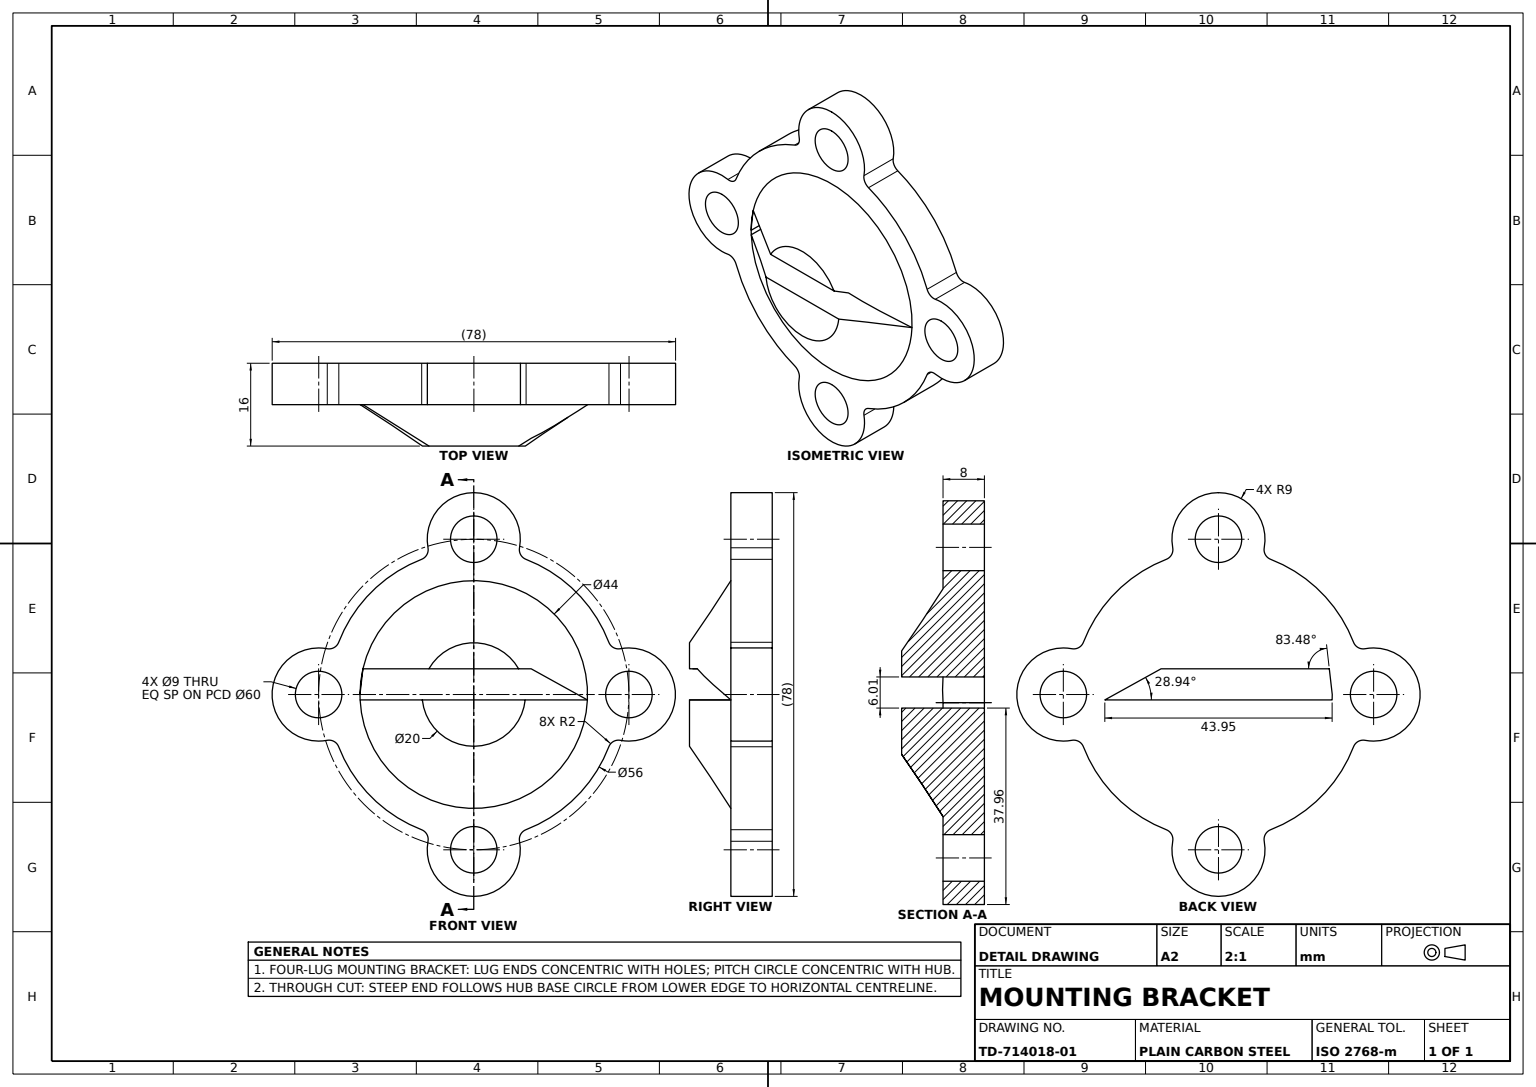
ISO-10303-21;
HEADER;
FILE_DESCRIPTION((''),'2;1');
FILE_NAME('','',(''),(''),'','','');
FILE_SCHEMA(('AUTOMOTIVE_DESIGN'));
ENDSEC;
DATA;
#1=APPLICATION_CONTEXT('');
#2=PRODUCT_CONTEXT('',#1,'mechanical');
#3=PRODUCT('','','',(#2));
#4=PRODUCT_DEFINITION_FORMATION('','',#3);
#5=PRODUCT_DEFINITION_CONTEXT('',#1,'design');
#6=PRODUCT_DEFINITION('','',#4,#5);
#7=PRODUCT_DEFINITION_SHAPE('','',#6);
#8=(LENGTH_UNIT()NAMED_UNIT(*)SI_UNIT(.MILLI.,.METRE.));
#9=(NAMED_UNIT(*)PLANE_ANGLE_UNIT()SI_UNIT($,.RADIAN.));
#10=(NAMED_UNIT(*)SI_UNIT($,.STERADIAN.)SOLID_ANGLE_UNIT());
#11=UNCERTAINTY_MEASURE_WITH_UNIT(LENGTH_MEASURE(1.E-05),#8,'distance_accuracy_value','');
#12=(GEOMETRIC_REPRESENTATION_CONTEXT(3)GLOBAL_UNCERTAINTY_ASSIGNED_CONTEXT((#11))GLOBAL_UNIT_ASSIGNED_CONTEXT((#8,#9,#10))REPRESENTATION_CONTEXT('',''));
#13=CARTESIAN_POINT('',(30.,0.,9.));
#14=VERTEX_POINT('',#13);
#15=CARTESIAN_POINT('',(30.,0.,-9.));
#16=VERTEX_POINT('',#15);
#17=CARTESIAN_POINT('',(30.,0.,0.));
#18=DIRECTION('',(0.,1.,0.));
#19=DIRECTION('',(0.,0.,1.));
#20=AXIS2_PLACEMENT_3D('',#17,#18,#19);
#21=CIRCLE('',#20,9.);
#22=EDGE_CURVE('',#14,#16,#21,.T.);
#23=ORIENTED_EDGE('',*,*,#22,.T.);
#24=CARTESIAN_POINT('',(30.,8.,-9.));
#25=VERTEX_POINT('',#24);
#26=DIRECTION('',(0.,-1.,0.));
#27=VECTOR('',#26,1000.);
#28=LINE('',#24,#27);
#29=EDGE_CURVE('',#25,#16,#28,.T.);
#30=ORIENTED_EDGE('',*,*,#29,.F.);
#31=CARTESIAN_POINT('',(30.,8.,9.));
#32=VERTEX_POINT('',#31);
#33=CARTESIAN_POINT('',(30.,8.,0.));
#34=AXIS2_PLACEMENT_3D('',#33,#18,#19);
#35=CIRCLE('',#34,9.);
#36=EDGE_CURVE('',#32,#25,#35,.T.);
#37=ORIENTED_EDGE('',*,*,#36,.F.);
#38=LINE('',#31,#27);
#39=EDGE_CURVE('',#32,#14,#38,.T.);
#40=ORIENTED_EDGE('',*,*,#39,.T.);
#41=EDGE_LOOP('',(#23,#30,#37,#40));
#42=FACE_OUTER_BOUND('',#41,.T.);
#43=DIRECTION('',(0.,0.,-1.));
#44=AXIS2_PLACEMENT_3D('',#33,#26,#43);
#45=CYLINDRICAL_SURFACE('',#44,9.);
#46=ADVANCED_FACE('',(#42),#45,.T.);
#47=CARTESIAN_POINT('',(-28.35,8.,-8.847457));
#48=VERTEX_POINT('',#47);
#49=CARTESIAN_POINT('',(-30.,8.,-9.));
#50=VERTEX_POINT('',#49);
#51=CARTESIAN_POINT('',(-30.,8.,0.));
#52=AXIS2_PLACEMENT_3D('',#51,#18,#19);
#53=CIRCLE('',#52,9.);
#54=EDGE_CURVE('',#48,#50,#53,.T.);
#55=ORIENTED_EDGE('',*,*,#54,.F.);
#56=CARTESIAN_POINT('',(-28.35,0.,-8.847457));
#57=VERTEX_POINT('',#56);
#58=LINE('',#47,#27);
#59=EDGE_CURVE('',#48,#57,#58,.T.);
#60=ORIENTED_EDGE('',*,*,#59,.T.);
#61=CARTESIAN_POINT('',(-30.,0.,-9.));
#62=VERTEX_POINT('',#61);
#63=CARTESIAN_POINT('',(-30.,0.,0.));
#64=AXIS2_PLACEMENT_3D('',#63,#18,#19);
#65=CIRCLE('',#64,9.);
#66=EDGE_CURVE('',#57,#62,#65,.T.);
#67=ORIENTED_EDGE('',*,*,#66,.T.);
#68=LINE('',#49,#27);
#69=EDGE_CURVE('',#50,#62,#68,.T.);
#70=ORIENTED_EDGE('',*,*,#69,.F.);
#71=EDGE_LOOP('',(#55,#60,#67,#70));
#72=FACE_OUTER_BOUND('',#71,.T.);
#73=AXIS2_PLACEMENT_3D('',#51,#26,#43);
#74=CYLINDRICAL_SURFACE('',#73,9.);
#75=ADVANCED_FACE('',(#72),#74,.T.);
#76=CARTESIAN_POINT('',(-8.847457,8.,-28.35));
#77=VERTEX_POINT('',#76);
#78=CARTESIAN_POINT('',(-8.847457,0.,-28.35));
#79=VERTEX_POINT('',#78);
#80=LINE('',#76,#27);
#81=EDGE_CURVE('',#77,#79,#80,.T.);
#82=ORIENTED_EDGE('',*,*,#81,.F.);
#83=CARTESIAN_POINT('',(0.,8.,-39.));
#84=VERTEX_POINT('',#83);
#85=CARTESIAN_POINT('',(0.,8.,-30.));
#86=AXIS2_PLACEMENT_3D('',#85,#18,#19);
#87=CIRCLE('',#86,9.);
#88=EDGE_CURVE('',#84,#77,#87,.T.);
#89=ORIENTED_EDGE('',*,*,#88,.F.);
#90=CARTESIAN_POINT('',(0.,0.,-39.));
#91=VERTEX_POINT('',#90);
#92=LINE('',#83,#27);
#93=EDGE_CURVE('',#84,#91,#92,.T.);
#94=ORIENTED_EDGE('',*,*,#93,.T.);
#95=CARTESIAN_POINT('',(0.,0.,-30.));
#96=AXIS2_PLACEMENT_3D('',#95,#18,#19);
#97=CIRCLE('',#96,9.);
#98=EDGE_CURVE('',#91,#79,#97,.T.);
#99=ORIENTED_EDGE('',*,*,#98,.T.);
#100=EDGE_LOOP('',(#82,#89,#94,#99));
#101=FACE_OUTER_BOUND('',#100,.T.);
#102=AXIS2_PLACEMENT_3D('',#85,#26,#43);
#103=CYLINDRICAL_SURFACE('',#102,9.);
#104=ADVANCED_FACE('',(#101),#103,.T.);
#105=CARTESIAN_POINT('',(-10.092655,8.,26.117778));
#106=VERTEX_POINT('',#105);
#107=CARTESIAN_POINT('',(-10.092655,0.,26.117778));
#108=VERTEX_POINT('',#107);
#109=LINE('',#105,#27);
#110=EDGE_CURVE('',#106,#108,#109,.T.);
#111=ORIENTED_EDGE('',*,*,#110,.F.);
#112=CARTESIAN_POINT('',(-26.117778,8.,10.092655));
#113=VERTEX_POINT('',#112);
#114=CARTESIAN_POINT('',(0.,8.,0.));
#115=AXIS2_PLACEMENT_3D('',#114,#18,#19);
#116=CIRCLE('',#115,28.);
#117=EDGE_CURVE('',#113,#106,#116,.T.);
#118=ORIENTED_EDGE('',*,*,#117,.F.);
#119=CARTESIAN_POINT('',(-26.117778,0.,10.092655));
#120=VERTEX_POINT('',#119);
#121=LINE('',#112,#27);
#122=EDGE_CURVE('',#113,#120,#121,.T.);
#123=ORIENTED_EDGE('',*,*,#122,.T.);
#124=CARTESIAN_POINT('',(0.,0.,0.));
#125=AXIS2_PLACEMENT_3D('',#124,#18,#19);
#126=CIRCLE('',#125,28.);
#127=EDGE_CURVE('',#120,#108,#126,.T.);
#128=ORIENTED_EDGE('',*,*,#127,.T.);
#129=EDGE_LOOP('',(#111,#118,#123,#128));
#130=FACE_OUTER_BOUND('',#129,.T.);
#131=AXIS2_PLACEMENT_3D('',#114,#26,#43);
#132=CYLINDRICAL_SURFACE('',#131,28.);
#133=ADVANCED_FACE('',(#130),#132,.T.);
#134=CARTESIAN_POINT('',(26.117778,0.,10.092655));
#135=VERTEX_POINT('',#134);
#136=CARTESIAN_POINT('',(27.983333,0.,8.813559));
#137=VERTEX_POINT('',#136);
#138=CARTESIAN_POINT('',(27.983333,0.,10.813559));
#139=AXIS2_PLACEMENT_3D('',#138,#26,#43);
#140=CIRCLE('',#139,2.);
#141=EDGE_CURVE('',#135,#137,#140,.T.);
#142=ORIENTED_EDGE('',*,*,#141,.T.);
#143=CARTESIAN_POINT('',(27.983333,8.,8.813559));
#144=VERTEX_POINT('',#143);
#145=LINE('',#143,#27);
#146=EDGE_CURVE('',#144,#137,#145,.T.);
#147=ORIENTED_EDGE('',*,*,#146,.F.);
#148=CARTESIAN_POINT('',(26.117778,8.,10.092655));
#149=VERTEX_POINT('',#148);
#150=CARTESIAN_POINT('',(27.983333,8.,10.813559));
#151=AXIS2_PLACEMENT_3D('',#150,#26,#43);
#152=CIRCLE('',#151,2.);
#153=EDGE_CURVE('',#149,#144,#152,.T.);
#154=ORIENTED_EDGE('',*,*,#153,.F.);
#155=LINE('',#148,#27);
#156=EDGE_CURVE('',#149,#135,#155,.T.);
#157=ORIENTED_EDGE('',*,*,#156,.T.);
#158=EDGE_LOOP('',(#142,#147,#154,#157));
#159=FACE_OUTER_BOUND('',#158,.T.);
#160=CYLINDRICAL_SURFACE('',#151,2.);
#161=ADVANCED_FACE('',(#159),#160,.F.);
#162=CARTESIAN_POINT('',(30.,8.,4.5));
#163=VERTEX_POINT('',#162);
#164=CARTESIAN_POINT('',(30.,0.,4.5));
#165=VERTEX_POINT('',#164);
#166=LINE('',#162,#27);
#167=EDGE_CURVE('',#163,#165,#166,.T.);
#168=ORIENTED_EDGE('',*,*,#167,.T.);
#169=CARTESIAN_POINT('',(30.,0.,-4.5));
#170=VERTEX_POINT('',#169);
#171=CIRCLE('',#20,4.5);
#172=EDGE_CURVE('',#170,#165,#171,.T.);
#173=ORIENTED_EDGE('',*,*,#172,.F.);
#174=CARTESIAN_POINT('',(30.,8.,-4.5));
#175=VERTEX_POINT('',#174);
#176=LINE('',#174,#27);
#177=EDGE_CURVE('',#175,#170,#176,.T.);
#178=ORIENTED_EDGE('',*,*,#177,.F.);
#179=CIRCLE('',#34,4.5);
#180=EDGE_CURVE('',#175,#163,#179,.T.);
#181=ORIENTED_EDGE('',*,*,#180,.T.);
#182=EDGE_LOOP('',(#168,#173,#178,#181));
#183=FACE_OUTER_BOUND('',#182,.T.);
#184=CYLINDRICAL_SURFACE('',#44,4.5);
#185=ADVANCED_FACE('',(#183),#184,.F.);
#186=CARTESIAN_POINT('',(8.678873,16.,-4.967612));
#187=VERTEX_POINT('',#186);
#188=CARTESIAN_POINT('',(-8.678875,16.,-4.967612));
#189=VERTEX_POINT('',#188);
#190=CARTESIAN_POINT('',(0.,16.,0.));
#191=AXIS2_PLACEMENT_3D('',#190,#18,#19);
#192=CIRCLE('',#191,10.);
#193=EDGE_CURVE('',#187,#189,#192,.T.);
#194=ORIENTED_EDGE('',*,*,#193,.T.);
#195=CARTESIAN_POINT('',(0.,16.,-4.967612));
#196=DIRECTION('',(-1.,0.,0.));
#197=VECTOR('',#196,1000.);
#198=LINE('',#195,#197);
#199=EDGE_CURVE('',#187,#189,#198,.T.);
#200=ORIENTED_EDGE('',*,*,#199,.F.);
#201=EDGE_LOOP('',(#194,#200));
#202=FACE_OUTER_BOUND('',#201,.T.);
#203=PLANE('',#191);
#204=ADVANCED_FACE('',(#202),#203,.T.);
#205=CARTESIAN_POINT('',(-30.,8.,4.5));
#206=VERTEX_POINT('',#205);
#207=CARTESIAN_POINT('',(-30.,0.,4.5));
#208=VERTEX_POINT('',#207);
#209=LINE('',#205,#27);
#210=EDGE_CURVE('',#206,#208,#209,.T.);
#211=ORIENTED_EDGE('',*,*,#210,.F.);
#212=CARTESIAN_POINT('',(-30.,8.,-4.5));
#213=VERTEX_POINT('',#212);
#214=CIRCLE('',#52,4.5);
#215=EDGE_CURVE('',#206,#213,#214,.T.);
#216=ORIENTED_EDGE('',*,*,#215,.T.);
#217=CARTESIAN_POINT('',(-30.,0.,-4.5));
#218=VERTEX_POINT('',#217);
#219=LINE('',#212,#27);
#220=EDGE_CURVE('',#213,#218,#219,.T.);
#221=ORIENTED_EDGE('',*,*,#220,.T.);
#222=CIRCLE('',#64,4.5);
#223=EDGE_CURVE('',#208,#218,#222,.T.);
#224=ORIENTED_EDGE('',*,*,#223,.F.);
#225=EDGE_LOOP('',(#211,#216,#221,#224));
#226=FACE_OUTER_BOUND('',#225,.T.);
#227=CYLINDRICAL_SURFACE('',#73,4.5);
#228=ADVANCED_FACE('',(#226),#227,.F.);
#229=CARTESIAN_POINT('',(10.092655,8.,-26.117778));
#230=VERTEX_POINT('',#229);
#231=CARTESIAN_POINT('',(10.092655,0.,-26.117778));
#232=VERTEX_POINT('',#231);
#233=LINE('',#229,#27);
#234=EDGE_CURVE('',#230,#232,#233,.T.);
#235=ORIENTED_EDGE('',*,*,#234,.F.);
#236=CARTESIAN_POINT('',(26.117778,8.,-10.092655));
#237=VERTEX_POINT('',#236);
#238=EDGE_CURVE('',#237,#230,#116,.T.);
#239=ORIENTED_EDGE('',*,*,#238,.F.);
#240=CARTESIAN_POINT('',(26.117778,0.,-10.092655));
#241=VERTEX_POINT('',#240);
#242=LINE('',#236,#27);
#243=EDGE_CURVE('',#237,#241,#242,.T.);
#244=ORIENTED_EDGE('',*,*,#243,.T.);
#245=EDGE_CURVE('',#241,#232,#126,.T.);
#246=ORIENTED_EDGE('',*,*,#245,.T.);
#247=EDGE_LOOP('',(#235,#239,#244,#246));
#248=FACE_OUTER_BOUND('',#247,.T.);
#249=ADVANCED_FACE('',(#248),#132,.T.);
#250=CARTESIAN_POINT('',(0.,0.,34.5));
#251=VERTEX_POINT('',#250);
#252=CARTESIAN_POINT('',(0.,0.,25.5));
#253=VERTEX_POINT('',#252);
#254=CARTESIAN_POINT('',(0.,0.,30.));
#255=AXIS2_PLACEMENT_3D('',#254,#18,#19);
#256=CIRCLE('',#255,4.5);
#257=EDGE_CURVE('',#251,#253,#256,.T.);
#258=ORIENTED_EDGE('',*,*,#257,.F.);
#259=CARTESIAN_POINT('',(0.,8.,34.5));
#260=VERTEX_POINT('',#259);
#261=LINE('',#259,#27);
#262=EDGE_CURVE('',#260,#251,#261,.T.);
#263=ORIENTED_EDGE('',*,*,#262,.F.);
#264=CARTESIAN_POINT('',(0.,8.,25.5));
#265=VERTEX_POINT('',#264);
#266=CARTESIAN_POINT('',(0.,8.,30.));
#267=AXIS2_PLACEMENT_3D('',#266,#18,#19);
#268=CIRCLE('',#267,4.5);
#269=EDGE_CURVE('',#260,#265,#268,.T.);
#270=ORIENTED_EDGE('',*,*,#269,.T.);
#271=LINE('',#264,#27);
#272=EDGE_CURVE('',#265,#253,#271,.T.);
#273=ORIENTED_EDGE('',*,*,#272,.T.);
#274=EDGE_LOOP('',(#258,#263,#270,#273));
#275=FACE_OUTER_BOUND('',#274,.T.);
#276=AXIS2_PLACEMENT_3D('',#266,#26,#43);
#277=CYLINDRICAL_SURFACE('',#276,4.5);
#278=ADVANCED_FACE('',(#275),#277,.F.);
#279=CARTESIAN_POINT('',(-30.,8.,9.));
#280=VERTEX_POINT('',#279);
#281=EDGE_CURVE('',#50,#280,#53,.T.);
#282=ORIENTED_EDGE('',*,*,#281,.F.);
#283=ORIENTED_EDGE('',*,*,#69,.T.);
#284=CARTESIAN_POINT('',(-30.,0.,9.));
#285=VERTEX_POINT('',#284);
#286=EDGE_CURVE('',#62,#285,#65,.T.);
#287=ORIENTED_EDGE('',*,*,#286,.T.);
#288=LINE('',#279,#27);
#289=EDGE_CURVE('',#280,#285,#288,.T.);
#290=ORIENTED_EDGE('',*,*,#289,.F.);
#291=EDGE_LOOP('',(#282,#283,#287,#290));
#292=FACE_OUTER_BOUND('',#291,.T.);
#293=ADVANCED_FACE('',(#292),#74,.T.);
#294=CARTESIAN_POINT('',(0.,8.,-34.5));
#295=VERTEX_POINT('',#294);
#296=CARTESIAN_POINT('',(0.,8.,-25.5));
#297=VERTEX_POINT('',#296);
#298=CIRCLE('',#86,4.5);
#299=EDGE_CURVE('',#295,#297,#298,.T.);
#300=ORIENTED_EDGE('',*,*,#299,.T.);
#301=CARTESIAN_POINT('',(0.,0.,-25.5));
#302=VERTEX_POINT('',#301);
#303=LINE('',#296,#27);
#304=EDGE_CURVE('',#297,#302,#303,.T.);
#305=ORIENTED_EDGE('',*,*,#304,.T.);
#306=CARTESIAN_POINT('',(0.,0.,-34.5));
#307=VERTEX_POINT('',#306);
#308=CIRCLE('',#96,4.5);
#309=EDGE_CURVE('',#307,#302,#308,.T.);
#310=ORIENTED_EDGE('',*,*,#309,.F.);
#311=LINE('',#294,#27);
#312=EDGE_CURVE('',#295,#307,#311,.T.);
#313=ORIENTED_EDGE('',*,*,#312,.F.);
#314=EDGE_LOOP('',(#300,#305,#310,#313));
#315=FACE_OUTER_BOUND('',#314,.T.);
#316=CYLINDRICAL_SURFACE('',#102,4.5);
#317=ADVANCED_FACE('',(#315),#316,.F.);
#318=CARTESIAN_POINT('',(-9.945407,16.,1.043517));
#319=VERTEX_POINT('',#318);
#320=CARTESIAN_POINT('',(8.632899,16.,5.047085));
#321=VERTEX_POINT('',#320);
#322=EDGE_CURVE('',#319,#321,#192,.T.);
#323=ORIENTED_EDGE('',*,*,#322,.T.);
#324=CARTESIAN_POINT('',(9.945404,16.,1.043517));
#325=VERTEX_POINT('',#324);
#326=EDGE_CURVE('',#321,#325,#192,.T.);
#327=ORIENTED_EDGE('',*,*,#326,.T.);
#328=CARTESIAN_POINT('',(0.,16.,1.043517));
#329=DIRECTION('',(1.,0.,0.));
#330=VECTOR('',#329,1000.);
#331=LINE('',#328,#330);
#332=EDGE_CURVE('',#319,#325,#331,.T.);
#333=ORIENTED_EDGE('',*,*,#332,.F.);
#334=EDGE_LOOP('',(#323,#327,#333));
#335=FACE_OUTER_BOUND('',#334,.T.);
#336=ADVANCED_FACE('',(#335),#203,.T.);
#337=CARTESIAN_POINT('',(28.35,8.,-8.847457));
#338=VERTEX_POINT('',#337);
#339=CARTESIAN_POINT('',(28.35,0.,-8.847457));
#340=VERTEX_POINT('',#339);
#341=LINE('',#337,#27);
#342=EDGE_CURVE('',#338,#340,#341,.T.);
#343=ORIENTED_EDGE('',*,*,#342,.T.);
#344=CARTESIAN_POINT('',(27.983333,0.,-10.813559));
#345=AXIS2_PLACEMENT_3D('',#344,#26,#19);
#346=CIRCLE('',#345,2.);
#347=EDGE_CURVE('',#340,#241,#346,.T.);
#348=ORIENTED_EDGE('',*,*,#347,.T.);
#349=ORIENTED_EDGE('',*,*,#243,.F.);
#350=CARTESIAN_POINT('',(27.983333,8.,-10.813559));
#351=AXIS2_PLACEMENT_3D('',#350,#26,#19);
#352=CIRCLE('',#351,2.);
#353=EDGE_CURVE('',#338,#237,#352,.T.);
#354=ORIENTED_EDGE('',*,*,#353,.F.);
#355=EDGE_LOOP('',(#343,#348,#349,#354));
#356=FACE_OUTER_BOUND('',#355,.T.);
#357=AXIS2_PLACEMENT_3D('',#350,#26,#43);
#358=CYLINDRICAL_SURFACE('',#357,2.);
#359=ADVANCED_FACE('',(#356),#358,.F.);
#360=EDGE_CURVE('',#163,#175,#179,.T.);
#361=ORIENTED_EDGE('',*,*,#360,.T.);
#362=ORIENTED_EDGE('',*,*,#177,.T.);
#363=EDGE_CURVE('',#165,#170,#171,.T.);
#364=ORIENTED_EDGE('',*,*,#363,.F.);
#365=ORIENTED_EDGE('',*,*,#167,.F.);
#366=EDGE_LOOP('',(#361,#362,#364,#365));
#367=FACE_OUTER_BOUND('',#366,.T.);
#368=ADVANCED_FACE('',(#367),#184,.F.);
#369=ORIENTED_EDGE('',*,*,#234,.T.);
#370=CARTESIAN_POINT('',(8.847457,0.,-28.35));
#371=VERTEX_POINT('',#370);
#372=CARTESIAN_POINT('',(10.813559,0.,-27.983333));
#373=AXIS2_PLACEMENT_3D('',#372,#26,#19);
#374=CIRCLE('',#373,2.);
#375=EDGE_CURVE('',#232,#371,#374,.T.);
#376=ORIENTED_EDGE('',*,*,#375,.T.);
#377=CARTESIAN_POINT('',(8.847457,8.,-28.35));
#378=VERTEX_POINT('',#377);
#379=LINE('',#377,#27);
#380=EDGE_CURVE('',#378,#371,#379,.T.);
#381=ORIENTED_EDGE('',*,*,#380,.F.);
#382=CARTESIAN_POINT('',(10.813559,8.,-27.983333));
#383=AXIS2_PLACEMENT_3D('',#382,#26,#19);
#384=CIRCLE('',#383,2.);
#385=EDGE_CURVE('',#230,#378,#384,.T.);
#386=ORIENTED_EDGE('',*,*,#385,.F.);
#387=EDGE_LOOP('',(#369,#376,#381,#386));
#388=FACE_OUTER_BOUND('',#387,.T.);
#389=AXIS2_PLACEMENT_3D('',#382,#26,#43);
#390=CYLINDRICAL_SURFACE('',#389,2.);
#391=ADVANCED_FACE('',(#388),#390,.F.);
#392=EDGE_CURVE('',#218,#208,#222,.T.);
#393=ORIENTED_EDGE('',*,*,#392,.T.);
#394=ORIENTED_EDGE('',*,*,#223,.T.);
#395=EDGE_LOOP('',(#393,#394));
#396=FACE_BOUND('',#395,.T.);
#397=ORIENTED_EDGE('',*,*,#141,.F.);
#398=CARTESIAN_POINT('',(10.092655,0.,26.117778));
#399=VERTEX_POINT('',#398);
#400=EDGE_CURVE('',#399,#135,#126,.T.);
#401=ORIENTED_EDGE('',*,*,#400,.F.);
#402=CARTESIAN_POINT('',(8.847457,0.,28.35));
#403=VERTEX_POINT('',#402);
#404=CARTESIAN_POINT('',(10.813559,0.,27.983333));
#405=AXIS2_PLACEMENT_3D('',#404,#26,#43);
#406=CIRCLE('',#405,2.);
#407=EDGE_CURVE('',#403,#399,#406,.T.);
#408=ORIENTED_EDGE('',*,*,#407,.F.);
#409=CARTESIAN_POINT('',(-8.847457,0.,28.35));
#410=VERTEX_POINT('',#409);
#411=CIRCLE('',#255,9.);
#412=EDGE_CURVE('',#410,#403,#411,.T.);
#413=ORIENTED_EDGE('',*,*,#412,.F.);
#414=CARTESIAN_POINT('',(-10.813559,0.,27.983333));
#415=AXIS2_PLACEMENT_3D('',#414,#26,#43);
#416=CIRCLE('',#415,2.);
#417=EDGE_CURVE('',#108,#410,#416,.T.);
#418=ORIENTED_EDGE('',*,*,#417,.F.);
#419=ORIENTED_EDGE('',*,*,#127,.F.);
#420=CARTESIAN_POINT('',(-27.983333,0.,8.813559));
#421=VERTEX_POINT('',#420);
#422=CARTESIAN_POINT('',(-27.983333,0.,10.813559));
#423=AXIS2_PLACEMENT_3D('',#422,#26,#43);
#424=CIRCLE('',#423,2.);
#425=EDGE_CURVE('',#421,#120,#424,.T.);
#426=ORIENTED_EDGE('',*,*,#425,.F.);
#427=CARTESIAN_POINT('',(-28.35,0.,8.847457));
#428=VERTEX_POINT('',#427);
#429=EDGE_CURVE('',#428,#421,#424,.T.);
#430=ORIENTED_EDGE('',*,*,#429,.F.);
#431=EDGE_CURVE('',#285,#428,#65,.T.);
#432=ORIENTED_EDGE('',*,*,#431,.F.);
#433=ORIENTED_EDGE('',*,*,#286,.F.);
#434=ORIENTED_EDGE('',*,*,#66,.F.);
#435=CARTESIAN_POINT('',(-26.117778,0.,-10.092655));
#436=VERTEX_POINT('',#435);
#437=CARTESIAN_POINT('',(-27.983333,0.,-10.813559));
#438=AXIS2_PLACEMENT_3D('',#437,#26,#19);
#439=CIRCLE('',#438,2.);
#440=EDGE_CURVE('',#436,#57,#439,.T.);
#441=ORIENTED_EDGE('',*,*,#440,.F.);
#442=CARTESIAN_POINT('',(-10.092655,0.,-26.117778));
#443=VERTEX_POINT('',#442);
#444=EDGE_CURVE('',#443,#436,#126,.T.);
#445=ORIENTED_EDGE('',*,*,#444,.F.);
#446=CARTESIAN_POINT('',(-10.813559,0.,-27.983333));
#447=AXIS2_PLACEMENT_3D('',#446,#26,#19);
#448=CIRCLE('',#447,2.);
#449=EDGE_CURVE('',#79,#443,#448,.T.);
#450=ORIENTED_EDGE('',*,*,#449,.F.);
#451=ORIENTED_EDGE('',*,*,#98,.F.);
#452=EDGE_CURVE('',#371,#91,#97,.T.);
#453=ORIENTED_EDGE('',*,*,#452,.F.);
#454=ORIENTED_EDGE('',*,*,#375,.F.);
#455=ORIENTED_EDGE('',*,*,#245,.F.);
#456=ORIENTED_EDGE('',*,*,#347,.F.);
#457=EDGE_CURVE('',#16,#340,#21,.T.);
#458=ORIENTED_EDGE('',*,*,#457,.F.);
#459=ORIENTED_EDGE('',*,*,#22,.F.);
#460=CARTESIAN_POINT('',(28.35,0.,8.847457));
#461=VERTEX_POINT('',#460);
#462=EDGE_CURVE('',#461,#14,#21,.T.);
#463=ORIENTED_EDGE('',*,*,#462,.F.);
#464=EDGE_CURVE('',#137,#461,#140,.T.);
#465=ORIENTED_EDGE('',*,*,#464,.F.);
#466=EDGE_LOOP('',(#397,#401,#408,#413,#418,#419,#426,#430,#432,#433,#434,#441,#445,#450,#451,#453,#454,#455,#456,#458,#459,#463,#465));
#467=FACE_OUTER_BOUND('',#466,.T.);
#468=ORIENTED_EDGE('',*,*,#257,.T.);
#469=EDGE_CURVE('',#253,#251,#256,.T.);
#470=ORIENTED_EDGE('',*,*,#469,.T.);
#471=EDGE_LOOP('',(#468,#470));
#472=FACE_BOUND('',#471,.T.);
#473=CARTESIAN_POINT('',(11.101907,0.,-4.967612));
#474=VERTEX_POINT('',#473);
#475=CARTESIAN_POINT('',(-21.431818,0.,-4.967612));
#476=VERTEX_POINT('',#475);
#477=LINE('',#475,#197);
#478=EDGE_CURVE('',#474,#476,#477,.T.);
#479=ORIENTED_EDGE('',*,*,#478,.T.);
#480=CARTESIAN_POINT('',(-22.,0.,0.));
#481=VERTEX_POINT('',#480);
#482=DIRECTION('',(-0.113636364,0.,0.993522409));
#483=VECTOR('',#482,1000.);
#484=LINE('',#480,#483);
#485=EDGE_CURVE('',#476,#481,#484,.T.);
#486=ORIENTED_EDGE('',*,*,#485,.T.);
#487=CARTESIAN_POINT('',(-21.975238,0.,1.043517));
#488=VERTEX_POINT('',#487);
#489=DIRECTION('',(0.023722969,0.,0.999718571));
#490=VECTOR('',#489,1000.);
#491=LINE('',#487,#490);
#492=EDGE_CURVE('',#481,#488,#491,.T.);
#493=ORIENTED_EDGE('',*,*,#492,.T.);
#494=CARTESIAN_POINT('',(21.975238,0.,1.043517));
#495=VERTEX_POINT('',#494);
#496=LINE('',#494,#330);
#497=EDGE_CURVE('',#488,#495,#496,.T.);
#498=ORIENTED_EDGE('',*,*,#497,.T.);
#499=DIRECTION('',(-0.875167149,0.,-0.483820692));
#500=VECTOR('',#499,1000.);
#501=LINE('',#473,#500);
#502=EDGE_CURVE('',#495,#474,#501,.T.);
#503=ORIENTED_EDGE('',*,*,#502,.T.);
#504=EDGE_LOOP('',(#479,#486,#493,#498,#503));
#505=FACE_BOUND('',#504,.T.);
#506=ORIENTED_EDGE('',*,*,#309,.T.);
#507=EDGE_CURVE('',#302,#307,#308,.T.);
#508=ORIENTED_EDGE('',*,*,#507,.T.);
#509=EDGE_LOOP('',(#506,#508));
#510=FACE_BOUND('',#509,.T.);
#511=ORIENTED_EDGE('',*,*,#172,.T.);
#512=ORIENTED_EDGE('',*,*,#363,.T.);
#513=EDGE_LOOP('',(#511,#512));
#514=FACE_BOUND('',#513,.T.);
#515=CARTESIAN_POINT('',(-5.406779,0.,-28.991667));
#516=AXIS2_PLACEMENT_3D('',#515,#18,#19);
#517=PLANE('',#516);
#518=ADVANCED_FACE('',(#396,#467,#472,#505,#510,#514),#517,.F.);
#519=ORIENTED_EDGE('',*,*,#342,.F.);
#520=EDGE_CURVE('',#25,#338,#35,.T.);
#521=ORIENTED_EDGE('',*,*,#520,.F.);
#522=ORIENTED_EDGE('',*,*,#29,.T.);
#523=ORIENTED_EDGE('',*,*,#457,.T.);
#524=EDGE_LOOP('',(#519,#521,#522,#523));
#525=FACE_OUTER_BOUND('',#524,.T.);
#526=ADVANCED_FACE('',(#525),#45,.T.);
#527=ORIENTED_EDGE('',*,*,#429,.T.);
#528=CARTESIAN_POINT('',(-27.983333,8.,8.813559));
#529=VERTEX_POINT('',#528);
#530=LINE('',#528,#27);
#531=EDGE_CURVE('',#529,#421,#530,.T.);
#532=ORIENTED_EDGE('',*,*,#531,.F.);
#533=CARTESIAN_POINT('',(-28.35,8.,8.847457));
#534=VERTEX_POINT('',#533);
#535=CARTESIAN_POINT('',(-27.983333,8.,10.813559));
#536=AXIS2_PLACEMENT_3D('',#535,#26,#43);
#537=CIRCLE('',#536,2.);
#538=EDGE_CURVE('',#534,#529,#537,.T.);
#539=ORIENTED_EDGE('',*,*,#538,.F.);
#540=LINE('',#533,#27);
#541=EDGE_CURVE('',#534,#428,#540,.T.);
#542=ORIENTED_EDGE('',*,*,#541,.T.);
#543=EDGE_LOOP('',(#527,#532,#539,#542));
#544=FACE_OUTER_BOUND('',#543,.T.);
#545=CYLINDRICAL_SURFACE('',#536,2.);
#546=ADVANCED_FACE('',(#544),#545,.F.);
#547=CARTESIAN_POINT('',(-21.975238,8.,1.043517));
#548=VERTEX_POINT('',#547);
#549=CARTESIAN_POINT('',(-19.950624,9.303741,1.043517));
#550=CARTESIAN_POINT('',(-17.929405,10.612793,1.043517));
#551=CARTESIAN_POINT('',(-14.913271,12.600284,1.043517));
#552=CARTESIAN_POINT('',(-13.910544,13.266852,1.043517));
#553=CARTESIAN_POINT('',(-11.916145,14.616313,1.043517));
#554=CARTESIAN_POINT('',(-10.924071,15.298459,1.043517));
#555=B_SPLINE_CURVE_WITH_KNOTS('',3,(#547,#549,#550,#551,#552,#553,#554,#318),.UNSPECIFIED.,.F.,.F.,(4,2,2,4),(0.,0.007224165,0.010836247,0.01444833),.UNSPECIFIED.);
#556=EDGE_CURVE('',#548,#319,#555,.T.);
#557=ORIENTED_EDGE('',*,*,#556,.T.);
#558=ORIENTED_EDGE('',*,*,#332,.T.);
#559=CARTESIAN_POINT('',(21.975238,8.,1.043517));
#560=VERTEX_POINT('',#559);
#561=CARTESIAN_POINT('',(10.924077,15.298455,1.043517));
#562=CARTESIAN_POINT('',(11.916147,14.616311,1.043517));
#563=CARTESIAN_POINT('',(13.910532,13.26686,1.043517));
#564=CARTESIAN_POINT('',(14.913267,12.600287,1.043517));
#565=CARTESIAN_POINT('',(17.929396,10.612799,1.043517));
#566=CARTESIAN_POINT('',(19.950622,9.303742,1.043517));
#567=B_SPLINE_CURVE_WITH_KNOTS('',3,(#324,#561,#562,#563,#564,#565,#566,#559),.UNSPECIFIED.,.F.,.F.,(4,2,2,4),(0.,0.003611877,0.007223754,0.014447508),.UNSPECIFIED.);
#568=EDGE_CURVE('',#325,#560,#567,.T.);
#569=ORIENTED_EDGE('',*,*,#568,.T.);
#570=VECTOR('',#18,1000.);
#571=LINE('',#494,#570);
#572=EDGE_CURVE('',#495,#560,#571,.T.);
#573=ORIENTED_EDGE('',*,*,#572,.F.);
#574=ORIENTED_EDGE('',*,*,#497,.F.);
#575=LINE('',#487,#570);
#576=EDGE_CURVE('',#488,#548,#575,.T.);
#577=ORIENTED_EDGE('',*,*,#576,.T.);
#578=EDGE_LOOP('',(#557,#558,#569,#573,#574,#577));
#579=FACE_OUTER_BOUND('',#578,.T.);
#580=AXIS2_PLACEMENT_3D('',#494,#19,#329);
#581=PLANE('',#580);
#582=ADVANCED_FACE('',(#579),#581,.F.);
#583=CARTESIAN_POINT('',(8.847457,8.,28.35));
#584=VERTEX_POINT('',#583);
#585=CARTESIAN_POINT('',(10.092655,8.,26.117778));
#586=VERTEX_POINT('',#585);
#587=CARTESIAN_POINT('',(10.813559,8.,27.983333));
#588=AXIS2_PLACEMENT_3D('',#587,#26,#43);
#589=CIRCLE('',#588,2.);
#590=EDGE_CURVE('',#584,#586,#589,.T.);
#591=ORIENTED_EDGE('',*,*,#590,.F.);
#592=LINE('',#583,#27);
#593=EDGE_CURVE('',#584,#403,#592,.T.);
#594=ORIENTED_EDGE('',*,*,#593,.T.);
#595=ORIENTED_EDGE('',*,*,#407,.T.);
#596=LINE('',#585,#27);
#597=EDGE_CURVE('',#586,#399,#596,.T.);
#598=ORIENTED_EDGE('',*,*,#597,.F.);
#599=EDGE_LOOP('',(#591,#594,#595,#598));
#600=FACE_OUTER_BOUND('',#599,.T.);
#601=CYLINDRICAL_SURFACE('',#588,2.);
#602=ADVANCED_FACE('',(#600),#601,.F.);
#603=CARTESIAN_POINT('',(-26.117778,8.,-10.092655));
#604=VERTEX_POINT('',#603);
#605=CARTESIAN_POINT('',(-27.983333,8.,-10.813559));
#606=AXIS2_PLACEMENT_3D('',#605,#26,#19);
#607=CIRCLE('',#606,2.);
#608=EDGE_CURVE('',#604,#48,#607,.T.);
#609=ORIENTED_EDGE('',*,*,#608,.F.);
#610=LINE('',#603,#27);
#611=EDGE_CURVE('',#604,#436,#610,.T.);
#612=ORIENTED_EDGE('',*,*,#611,.T.);
#613=ORIENTED_EDGE('',*,*,#440,.T.);
#614=ORIENTED_EDGE('',*,*,#59,.F.);
#615=EDGE_LOOP('',(#609,#612,#613,#614));
#616=FACE_OUTER_BOUND('',#615,.T.);
#617=AXIS2_PLACEMENT_3D('',#605,#26,#43);
#618=CYLINDRICAL_SURFACE('',#617,2.);
#619=ADVANCED_FACE('',(#616),#618,.F.);
#620=ORIENTED_EDGE('',*,*,#81,.T.);
#621=ORIENTED_EDGE('',*,*,#449,.T.);
#622=CARTESIAN_POINT('',(-10.092655,8.,-26.117778));
#623=VERTEX_POINT('',#622);
#624=LINE('',#622,#27);
#625=EDGE_CURVE('',#623,#443,#624,.T.);
#626=ORIENTED_EDGE('',*,*,#625,.F.);
#627=CARTESIAN_POINT('',(-10.813559,8.,-27.983333));
#628=AXIS2_PLACEMENT_3D('',#627,#26,#19);
#629=CIRCLE('',#628,2.);
#630=EDGE_CURVE('',#77,#623,#629,.T.);
#631=ORIENTED_EDGE('',*,*,#630,.F.);
#632=EDGE_LOOP('',(#620,#621,#626,#631));
#633=FACE_OUTER_BOUND('',#632,.T.);
#634=AXIS2_PLACEMENT_3D('',#627,#26,#43);
#635=CYLINDRICAL_SURFACE('',#634,2.);
#636=ADVANCED_FACE('',(#633),#635,.F.);
#637=ORIENTED_EDGE('',*,*,#576,.F.);
#638=ORIENTED_EDGE('',*,*,#492,.F.);
#639=CARTESIAN_POINT('',(-22.,8.,0.));
#640=VERTEX_POINT('',#639);
#641=LINE('',#480,#570);
#642=EDGE_CURVE('',#481,#640,#641,.T.);
#643=ORIENTED_EDGE('',*,*,#642,.T.);
#644=LINE('',#547,#490);
#645=EDGE_CURVE('',#640,#548,#644,.T.);
#646=ORIENTED_EDGE('',*,*,#645,.T.);
#647=EDGE_LOOP('',(#637,#638,#643,#646));
#648=FACE_OUTER_BOUND('',#647,.T.);
#649=DIRECTION('',(-0.999718571,0.,0.023722969));
#650=AXIS2_PLACEMENT_3D('',#487,#649,#489);
#651=PLANE('',#650);
#652=ADVANCED_FACE('',(#648),#651,.F.);
#653=ORIENTED_EDGE('',*,*,#444,.T.);
#654=ORIENTED_EDGE('',*,*,#611,.F.);
#655=EDGE_CURVE('',#623,#604,#116,.T.);
#656=ORIENTED_EDGE('',*,*,#655,.F.);
#657=ORIENTED_EDGE('',*,*,#625,.T.);
#658=EDGE_LOOP('',(#653,#654,#656,#657));
#659=FACE_OUTER_BOUND('',#658,.T.);
#660=ADVANCED_FACE('',(#659),#132,.T.);
#661=ORIENTED_EDGE('',*,*,#322,.F.);
#662=ORIENTED_EDGE('',*,*,#556,.F.);
#663=CARTESIAN_POINT('',(15.07011,8.,16.027844));
#664=VERTEX_POINT('',#663);
#665=CIRCLE('',#115,22.);
#666=EDGE_CURVE('',#548,#664,#665,.T.);
#667=ORIENTED_EDGE('',*,*,#666,.T.);
#668=B_SPLINE_CURVE_WITH_KNOTS('',1,(#663,#320),.UNSPECIFIED.,.F.,.F.,(2,2),(0.,1.),.UNSPECIFIED.);
#669=EDGE_CURVE('',#664,#321,#668,.T.);
#670=ORIENTED_EDGE('',*,*,#669,.T.);
#671=EDGE_LOOP('',(#661,#662,#667,#670));
#672=FACE_OUTER_BOUND('',#671,.T.);
#673=CARTESIAN_POINT('',(8.632899,16.,5.047084));
#674=CARTESIAN_POINT('',(47.125798,8.,-14.112376));
#675=CARTESIAN_POINT('',(18.727067,16.,-12.218713));
#676=CARTESIAN_POINT('',(16.985578,8.,-46.168064));
#677=CARTESIAN_POINT('',(1.46127,16.,-22.312882));
#678=CARTESIAN_POINT('',(-15.07011,8.,-16.027844));
#679=CARTESIAN_POINT('',(-8.632899,16.,-5.047084));
#680=CARTESIAN_POINT('',(-47.125798,8.,14.112376));
#681=CARTESIAN_POINT('',(-18.727067,16.,12.218713));
#682=CARTESIAN_POINT('',(-16.985578,8.,46.168064));
#683=CARTESIAN_POINT('',(-1.46127,16.,22.312882));
#684=(BOUNDED_SURFACE()B_SPLINE_SURFACE(3,1,((#663,#673),(#674,#675),(#676,#677),(#678,#679),(#680,#681),(#682,#683),(#663,#673)),.UNSPECIFIED.,.T.,.F.,.T.)B_SPLINE_SURFACE_WITH_KNOTS((4,3,4),(2,2),(0.,0.5,1.),(0.,1.),.UNSPECIFIED.)GEOMETRIC_REPRESENTATION_ITEM()RATIONAL_B_SPLINE_SURFACE(((1.,1.),(0.333333333,0.333333333),(0.333333333,0.333333333),(1.,1.),(0.333333333,0.333333333),(0.333333333,0.333333333),(1.,1.)))REPRESENTATION_ITEM('')SURFACE());
#685=ADVANCED_FACE('',(#672),#684,.T.);
#686=CARTESIAN_POINT('',(28.35,8.,8.847457));
#687=VERTEX_POINT('',#686);
#688=EDGE_CURVE('',#144,#687,#152,.T.);
#689=ORIENTED_EDGE('',*,*,#688,.F.);
#690=ORIENTED_EDGE('',*,*,#146,.T.);
#691=ORIENTED_EDGE('',*,*,#464,.T.);
#692=LINE('',#686,#27);
#693=EDGE_CURVE('',#687,#461,#692,.T.);
#694=ORIENTED_EDGE('',*,*,#693,.F.);
#695=EDGE_LOOP('',(#689,#690,#691,#694));
#696=FACE_OUTER_BOUND('',#695,.T.);
#697=ADVANCED_FACE('',(#696),#160,.F.);
#698=ORIENTED_EDGE('',*,*,#425,.T.);
#699=ORIENTED_EDGE('',*,*,#122,.F.);
#700=EDGE_CURVE('',#529,#113,#537,.T.);
#701=ORIENTED_EDGE('',*,*,#700,.F.);
#702=ORIENTED_EDGE('',*,*,#531,.T.);
#703=EDGE_LOOP('',(#698,#699,#701,#702));
#704=FACE_OUTER_BOUND('',#703,.T.);
#705=ADVANCED_FACE('',(#704),#545,.F.);
#706=ORIENTED_EDGE('',*,*,#642,.F.);
#707=ORIENTED_EDGE('',*,*,#485,.F.);
#708=CARTESIAN_POINT('',(-21.431818,8.,-4.967612));
#709=VERTEX_POINT('',#708);
#710=LINE('',#475,#570);
#711=EDGE_CURVE('',#476,#709,#710,.T.);
#712=ORIENTED_EDGE('',*,*,#711,.T.);
#713=CARTESIAN_POINT('',(-21.621212,8.122097,-3.311741));
#714=CARTESIAN_POINT('',(-21.810606,8.122097,-1.655871));
#715=B_SPLINE_CURVE_WITH_KNOTS('',3,(#708,#713,#714,#639),.UNSPECIFIED.,.F.,.F.,(4,4),(0.,0.005),.UNSPECIFIED.);
#716=EDGE_CURVE('',#709,#640,#715,.T.);
#717=ORIENTED_EDGE('',*,*,#716,.T.);
#718=EDGE_LOOP('',(#706,#707,#712,#717));
#719=FACE_OUTER_BOUND('',#718,.T.);
#720=DIRECTION('',(-0.993522409,0.,-0.113636364));
#721=AXIS2_PLACEMENT_3D('',#480,#720,#482);
#722=PLANE('',#721);
#723=ADVANCED_FACE('',(#719),#722,.F.);
#724=ORIENTED_EDGE('',*,*,#469,.F.);
#725=ORIENTED_EDGE('',*,*,#272,.F.);
#726=EDGE_CURVE('',#265,#260,#268,.T.);
#727=ORIENTED_EDGE('',*,*,#726,.T.);
#728=ORIENTED_EDGE('',*,*,#262,.T.);
#729=EDGE_LOOP('',(#724,#725,#727,#728));
#730=FACE_OUTER_BOUND('',#729,.T.);
#731=ADVANCED_FACE('',(#730),#277,.F.);
#732=ORIENTED_EDGE('',*,*,#462,.T.);
#733=ORIENTED_EDGE('',*,*,#39,.F.);
#734=EDGE_CURVE('',#687,#32,#35,.T.);
#735=ORIENTED_EDGE('',*,*,#734,.F.);
#736=ORIENTED_EDGE('',*,*,#693,.T.);
#737=EDGE_LOOP('',(#732,#733,#735,#736));
#738=FACE_OUTER_BOUND('',#737,.T.);
#739=ADVANCED_FACE('',(#738),#45,.T.);
#740=ORIENTED_EDGE('',*,*,#289,.T.);
#741=ORIENTED_EDGE('',*,*,#431,.T.);
#742=ORIENTED_EDGE('',*,*,#541,.F.);
#743=EDGE_CURVE('',#280,#534,#53,.T.);
#744=ORIENTED_EDGE('',*,*,#743,.F.);
#745=EDGE_LOOP('',(#740,#741,#742,#744));
#746=FACE_OUTER_BOUND('',#745,.T.);
#747=ADVANCED_FACE('',(#746),#74,.T.);
#748=ORIENTED_EDGE('',*,*,#417,.T.);
#749=CARTESIAN_POINT('',(-8.847457,8.,28.35));
#750=VERTEX_POINT('',#749);
#751=LINE('',#749,#27);
#752=EDGE_CURVE('',#750,#410,#751,.T.);
#753=ORIENTED_EDGE('',*,*,#752,.F.);
#754=CARTESIAN_POINT('',(-10.813559,8.,27.983333));
#755=AXIS2_PLACEMENT_3D('',#754,#26,#43);
#756=CIRCLE('',#755,2.);
#757=EDGE_CURVE('',#106,#750,#756,.T.);
#758=ORIENTED_EDGE('',*,*,#757,.F.);
#759=ORIENTED_EDGE('',*,*,#110,.T.);
#760=EDGE_LOOP('',(#748,#753,#758,#759));
#761=FACE_OUTER_BOUND('',#760,.T.);
#762=CYLINDRICAL_SURFACE('',#755,2.);
#763=ADVANCED_FACE('',(#761),#762,.F.);
#764=ORIENTED_EDGE('',*,*,#93,.F.);
#765=EDGE_CURVE('',#378,#84,#87,.T.);
#766=ORIENTED_EDGE('',*,*,#765,.F.);
#767=ORIENTED_EDGE('',*,*,#380,.T.);
#768=ORIENTED_EDGE('',*,*,#452,.T.);
#769=EDGE_LOOP('',(#764,#766,#767,#768));
#770=FACE_OUTER_BOUND('',#769,.T.);
#771=ADVANCED_FACE('',(#770),#103,.T.);
#772=ORIENTED_EDGE('',*,*,#392,.F.);
#773=ORIENTED_EDGE('',*,*,#220,.F.);
#774=EDGE_CURVE('',#213,#206,#214,.T.);
#775=ORIENTED_EDGE('',*,*,#774,.T.);
#776=ORIENTED_EDGE('',*,*,#210,.T.);
#777=EDGE_LOOP('',(#772,#773,#775,#776));
#778=FACE_OUTER_BOUND('',#777,.T.);
#779=ADVANCED_FACE('',(#778),#227,.F.);
#780=EDGE_CURVE('',#586,#149,#116,.T.);
#781=ORIENTED_EDGE('',*,*,#780,.F.);
#782=ORIENTED_EDGE('',*,*,#597,.T.);
#783=ORIENTED_EDGE('',*,*,#400,.T.);
#784=ORIENTED_EDGE('',*,*,#156,.F.);
#785=EDGE_LOOP('',(#781,#782,#783,#784));
#786=FACE_OUTER_BOUND('',#785,.T.);
#787=ADVANCED_FACE('',(#786),#132,.T.);
#788=ORIENTED_EDGE('',*,*,#669,.F.);
#789=EDGE_CURVE('',#664,#560,#665,.T.);
#790=ORIENTED_EDGE('',*,*,#789,.T.);
#791=ORIENTED_EDGE('',*,*,#568,.F.);
#792=ORIENTED_EDGE('',*,*,#326,.F.);
#793=EDGE_LOOP('',(#788,#790,#791,#792));
#794=FACE_OUTER_BOUND('',#793,.T.);
#795=(BOUNDED_SURFACE()B_SPLINE_SURFACE(3,1,((#663,#673),(#674,#675),(#676,#677),(#678,#679),(#680,#681),(#682,#683),(#663,#673)),.UNSPECIFIED.,.T.,.F.,.F.)B_SPLINE_SURFACE_WITH_KNOTS((4,3,4),(2,2),(0.,0.5,1.),(0.,1.),.UNSPECIFIED.)GEOMETRIC_REPRESENTATION_ITEM()RATIONAL_B_SPLINE_SURFACE(((1.,1.),(0.333333333,0.333333333),(0.333333333,0.333333333),(1.,1.),(0.333333333,0.333333333),(0.333333333,0.333333333),(1.,1.)))REPRESENTATION_ITEM('')SURFACE());
#796=ADVANCED_FACE('',(#794),#795,.T.);
#797=CARTESIAN_POINT('',(-9.887139,15.244174,-4.967612));
#798=CARTESIAN_POINT('',(-11.094795,14.487372,-4.967612));
#799=CARTESIAN_POINT('',(-12.302255,13.730258,-4.967612));
#800=CARTESIAN_POINT('',(-13.509715,12.973144,-4.967612));
#801=CARTESIAN_POINT('',(-14.716952,12.215673,-4.967612));
#802=CARTESIAN_POINT('',(-15.924088,11.458044,-4.967612));
#803=CARTESIAN_POINT('',(-17.760186,10.305662,-4.967612));
#804=CARTESIAN_POINT('',(-19.596048,9.152904,-4.967612));
#805=B_SPLINE_CURVE_WITH_KNOTS('',3,(#188,#797,#798,#799,#800,#801,#802,#803,#804,#708),.UNSPECIFIED.,.F.,.F.,(4,3,3,4),(0.,0.004275586,0.00855117,0.015054489),.UNSPECIFIED.);
#806=EDGE_CURVE('',#189,#709,#805,.T.);
#807=ORIENTED_EDGE('',*,*,#806,.F.);
#808=ORIENTED_EDGE('',*,*,#193,.F.);
#809=CARTESIAN_POINT('',(11.101907,14.482721,-4.967612));
#810=VERTEX_POINT('',#809);
#811=CARTESIAN_POINT('',(10.294412,14.988773,-4.967612));
#812=CARTESIAN_POINT('',(9.486785,15.494614,-4.967612));
#813=B_SPLINE_CURVE_WITH_KNOTS('',3,(#809,#811,#812,#186),.UNSPECIFIED.,.F.,.F.,(4,4),(0.,0.002858886),.UNSPECIFIED.);
#814=EDGE_CURVE('',#810,#187,#813,.T.);
#815=ORIENTED_EDGE('',*,*,#814,.F.);
#816=CARTESIAN_POINT('',(20.204247,9.17036,0.064456));
#817=CARTESIAN_POINT('',(18.423879,10.322932,-0.919789));
#818=CARTESIAN_POINT('',(15.718446,11.976796,-2.41544));
#819=CARTESIAN_POINT('',(14.811025,12.515009,-2.917091));
#820=CARTESIAN_POINT('',(12.975985,13.544358,-3.931561));
#821=CARTESIAN_POINT('',(12.048655,14.036168,-4.444219));
#822=B_SPLINE_CURVE_WITH_KNOTS('',3,(#559,#816,#817,#818,#819,#820,#821,#809),.UNSPECIFIED.,.F.,.F.,(4,2,2,4),(0.,0.007012521,0.010518782,0.014025042),.UNSPECIFIED.);
#823=EDGE_CURVE('',#560,#810,#822,.T.);
#824=ORIENTED_EDGE('',*,*,#823,.F.);
#825=EDGE_CURVE('',#560,#709,#665,.T.);
#826=ORIENTED_EDGE('',*,*,#825,.T.);
#827=EDGE_LOOP('',(#807,#808,#815,#824,#826));
#828=FACE_OUTER_BOUND('',#827,.T.);
#829=ADVANCED_FACE('',(#828),#795,.T.);
#830=ORIENTED_EDGE('',*,*,#412,.T.);
#831=ORIENTED_EDGE('',*,*,#593,.F.);
#832=CIRCLE('',#267,9.);
#833=EDGE_CURVE('',#750,#584,#832,.T.);
#834=ORIENTED_EDGE('',*,*,#833,.F.);
#835=ORIENTED_EDGE('',*,*,#752,.T.);
#836=EDGE_LOOP('',(#830,#831,#834,#835));
#837=FACE_OUTER_BOUND('',#836,.T.);
#838=CYLINDRICAL_SURFACE('',#276,9.);
#839=ADVANCED_FACE('',(#837),#838,.T.);
#840=ORIENTED_EDGE('',*,*,#304,.F.);
#841=EDGE_CURVE('',#297,#295,#298,.T.);
#842=ORIENTED_EDGE('',*,*,#841,.T.);
#843=ORIENTED_EDGE('',*,*,#312,.T.);
#844=ORIENTED_EDGE('',*,*,#507,.F.);
#845=EDGE_LOOP('',(#840,#842,#843,#844));
#846=FACE_OUTER_BOUND('',#845,.T.);
#847=ADVANCED_FACE('',(#846),#316,.F.);
#848=ORIENTED_EDGE('',*,*,#117,.T.);
#849=ORIENTED_EDGE('',*,*,#757,.T.);
#850=ORIENTED_EDGE('',*,*,#833,.T.);
#851=ORIENTED_EDGE('',*,*,#590,.T.);
#852=ORIENTED_EDGE('',*,*,#780,.T.);
#853=ORIENTED_EDGE('',*,*,#153,.T.);
#854=ORIENTED_EDGE('',*,*,#688,.T.);
#855=ORIENTED_EDGE('',*,*,#734,.T.);
#856=ORIENTED_EDGE('',*,*,#36,.T.);
#857=ORIENTED_EDGE('',*,*,#520,.T.);
#858=ORIENTED_EDGE('',*,*,#353,.T.);
#859=ORIENTED_EDGE('',*,*,#238,.T.);
#860=ORIENTED_EDGE('',*,*,#385,.T.);
#861=ORIENTED_EDGE('',*,*,#765,.T.);
#862=ORIENTED_EDGE('',*,*,#88,.T.);
#863=ORIENTED_EDGE('',*,*,#630,.T.);
#864=ORIENTED_EDGE('',*,*,#655,.T.);
#865=ORIENTED_EDGE('',*,*,#608,.T.);
#866=ORIENTED_EDGE('',*,*,#54,.T.);
#867=ORIENTED_EDGE('',*,*,#281,.T.);
#868=ORIENTED_EDGE('',*,*,#743,.T.);
#869=ORIENTED_EDGE('',*,*,#538,.T.);
#870=ORIENTED_EDGE('',*,*,#700,.T.);
#871=EDGE_LOOP('',(#848,#849,#850,#851,#852,#853,#854,#855,#856,#857,#858,#859,#860,#861,#862,#863,#864,#865,#866,#867,#868,#869,#870));
#872=FACE_OUTER_BOUND('',#871,.T.);
#873=ORIENTED_EDGE('',*,*,#360,.F.);
#874=ORIENTED_EDGE('',*,*,#180,.F.);
#875=EDGE_LOOP('',(#873,#874));
#876=FACE_BOUND('',#875,.T.);
#877=ORIENTED_EDGE('',*,*,#215,.F.);
#878=ORIENTED_EDGE('',*,*,#774,.F.);
#879=EDGE_LOOP('',(#877,#878));
#880=FACE_BOUND('',#879,.T.);
#881=ORIENTED_EDGE('',*,*,#299,.F.);
#882=ORIENTED_EDGE('',*,*,#841,.F.);
#883=EDGE_LOOP('',(#881,#882));
#884=FACE_BOUND('',#883,.T.);
#885=ORIENTED_EDGE('',*,*,#789,.F.);
#886=ORIENTED_EDGE('',*,*,#666,.F.);
#887=ORIENTED_EDGE('',*,*,#645,.F.);
#888=EDGE_CURVE('',#709,#640,#665,.T.);
#889=ORIENTED_EDGE('',*,*,#888,.F.);
#890=ORIENTED_EDGE('',*,*,#825,.F.);
#891=EDGE_LOOP('',(#885,#886,#887,#889,#890));
#892=FACE_BOUND('',#891,.T.);
#893=ORIENTED_EDGE('',*,*,#726,.F.);
#894=ORIENTED_EDGE('',*,*,#269,.F.);
#895=EDGE_LOOP('',(#893,#894));
#896=FACE_BOUND('',#895,.T.);
#897=CARTESIAN_POINT('',(-5.406779,8.,-28.991667));
#898=AXIS2_PLACEMENT_3D('',#897,#18,#19);
#899=PLANE('',#898);
#900=ADVANCED_FACE('',(#872,#876,#880,#884,#892,#896),#899,.T.);
#901=ORIENTED_EDGE('',*,*,#814,.T.);
#902=ORIENTED_EDGE('',*,*,#199,.T.);
#903=ORIENTED_EDGE('',*,*,#806,.T.);
#904=ORIENTED_EDGE('',*,*,#711,.F.);
#905=ORIENTED_EDGE('',*,*,#478,.F.);
#906=LINE('',#473,#570);
#907=EDGE_CURVE('',#474,#810,#906,.T.);
#908=ORIENTED_EDGE('',*,*,#907,.T.);
#909=EDGE_LOOP('',(#901,#902,#903,#904,#905,#908));
#910=FACE_OUTER_BOUND('',#909,.T.);
#911=AXIS2_PLACEMENT_3D('',#475,#43,#196);
#912=PLANE('',#911);
#913=ADVANCED_FACE('',(#910),#912,.F.);
#914=ORIENTED_EDGE('',*,*,#502,.F.);
#915=ORIENTED_EDGE('',*,*,#572,.T.);
#916=ORIENTED_EDGE('',*,*,#823,.T.);
#917=ORIENTED_EDGE('',*,*,#907,.F.);
#918=EDGE_LOOP('',(#914,#915,#916,#917));
#919=FACE_OUTER_BOUND('',#918,.T.);
#920=DIRECTION('',(0.483820692,0.,-0.875167149));
#921=AXIS2_PLACEMENT_3D('',#473,#920,#499);
#922=PLANE('',#921);
#923=ADVANCED_FACE('',(#919),#922,.F.);
#924=ORIENTED_EDGE('',*,*,#888,.T.);
#925=ORIENTED_EDGE('',*,*,#716,.F.);
#926=EDGE_LOOP('',(#924,#925));
#927=FACE_OUTER_BOUND('',#926,.T.);
#928=ADVANCED_FACE('',(#927),#795,.T.);
#929=CLOSED_SHELL('',(#46,#75,#104,#133,#161,#185,#204,#228,#249,#278,#293,#317,#336,#359,#368,#391,#518,#526,#546,#582,#602,#619,#636,#652,#660,#685,#697,#705,#723,#731,#739,#747,#763,#771,#779,#787,#796,#829,#839,#847,#900,#913,#923,#928));
#930=MANIFOLD_SOLID_BREP('',#929);
#931=ADVANCED_BREP_SHAPE_REPRESENTATION('',(#930),#12);
#932=SHAPE_DEFINITION_REPRESENTATION(#7,#931);
ENDSEC;
END-ISO-10303-21;
